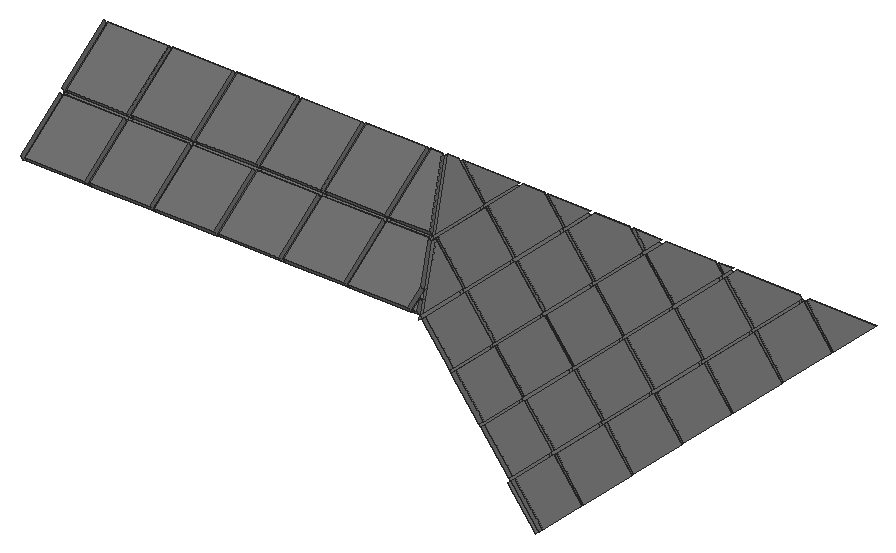
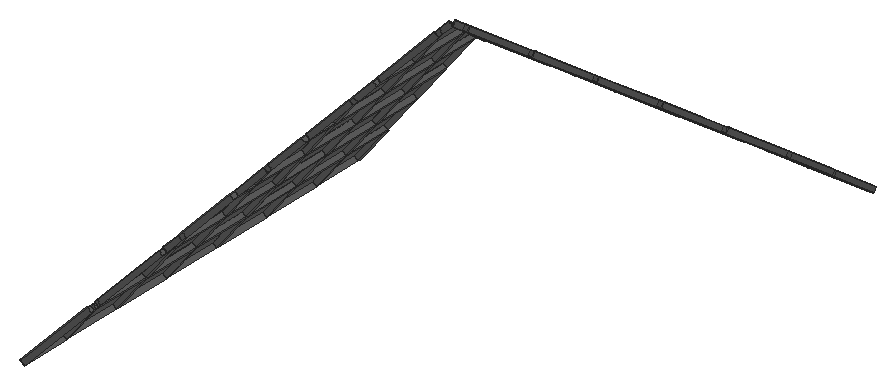
# SketchUp Ruby script. Lengths in inches.
U = 1.inch
M = Sketchup.active_model
def pt(a) = Geom::Point3d.new(a.map { |v| v * U })
def face(e, loops, mat)
  f = e.add_face(loops[0].map { |a| pt(a) })
  loops[1..].each { |l| e.add_face(l.map { |a| pt(a) }).erase! }
  f.material = f.back_material = mat if mat
  f
end
# faces: each face lists its corners as indices into pts; further lists are holes
def faces(e, pts, list, mat = nil) = list.each { |f| face(e, (f[0].is_a?(Array) ? f : [f]).map { |l| l.map { |i| pts[i] } }, mat) }
# xy, xz, yz: faces in a plane at the given z, y or x. An outline is a flat list of corners, or four numbers for a rectangle; further outlines are holes
def ring(l) = l.size == 4 ? [[l[0], l[1]], [l[2], l[1]], [l[2], l[3]], [l[0], l[3]]] : l.each_slice(2).to_a
def flat(e, list, mat, &to3) = list.each { |f| face(e, (f[0].is_a?(Array) ? f : [f]).map { |l| ring(l).map { |u, v| to3.(u, v) } }, mat) }
def xy(e, z, list, mat = nil) = flat(e, list, mat) { |x, y| [x, y, z] }
def xz(e, y, list, mat = nil) = flat(e, list, mat) { |x, z| [x, y, z] }
def yz(e, x, list, mat = nil) = flat(e, list, mat) { |y, z| [x, y, z] }
def lines(e, pts, list) = list.each { |a, b| e.add_line(pt(pts[a]), pt(pts[b])) }
# prism: a flat outline (further loops are holes) pulled along v
def prism(e, loops, v, mat = nil)
  f = face(e, loops, mat); d = Geom::Vector3d.new(v.map { |x| x * U })
  f.pushpull(f.normal.samedirection?(d) ? d.length : -d.length)
end
def box(e, o, s, mat = nil) = prism(e, [[o, [o[0] + s[0], o[1], o[2]], [o[0] + s[0], o[1] + s[1], o[2]], [o[0], o[1] + s[1], o[2]]]], [0, 0, s[2]], mat)
def at(x, y, z, deg = 0) = Geom::Transformation.translation(pt([x, y, z])) * Geom::Transformation.rotation(ORIGIN, Z_AXIS, deg.degrees)
def axes(o, x, y, z) = Geom::Transformation.new([*x, 0, *y, 0, *z, 0, *pt(o).to_a, 1])
def part(name) = M.definitions.add(name)
# library, detail: a bought-in or finely detailed component or shape, given as its bounding box
def library(name, o, s) = part(name).tap { |d| box(d.entities, o, s) }
def detail(e, o, s) = box(e.add_group.entities, o, s)
def put(e, d, t, mat = nil) = e.add_instance(d, t).tap { |i| i.material = mat if mat }
def group(e, t, mat = nil) = e.add_group.tap { |g| g.transformation = t; g.material = mat if mat }.entities
root = M.entities
M.materials.add("[Color M05]").color = [114, 114, 114]
xz(root,415.43,[[759.6,444.64,761.18,445.87,750.86,459.15,749.28,457.92],[748.6,458.81,750.18,460.04,739.86,473.32,738.28,472.1],[737.59,472.98,739.17,474.21,728.85,487.49,727.27,486.27],[726.58,487.15,728.16,488.38,717.84,501.67,716.26,500.4375]],"[Color M05]")
xz(root,433.59,[[759.6,444.64,749.28,457.92,750.86,459.15,761.18,445.87],[748.6,458.81,738.28,472.1,739.86,473.32,750.18,460.04],[737.59,472.98,727.27,486.27,728.85,487.49,739.17,474.21],[726.58,487.15,716.26,500.4375,717.84,501.67,728.16,488.38],[715.58,501.32,705.26,514.61,706.84,515.84,717.16,502.55]],"[Color M05]")
xz(root,434.8,[[759.6,444.64,761.18,445.87,750.86,459.15,749.28,457.92],[748.6,458.81,750.18,460.04,739.86,473.32,738.28,472.1],[737.59,472.98,739.17,474.21,728.85,487.49,727.27,486.27],[726.58,487.15,728.16,488.38,717.84,501.67,716.26,500.4375],[715.58,501.32,717.16,502.55,706.84,515.84,705.26,514.61]],"[Color M05]")
xz(root,456.8,[[759.6,444.64,749.28,457.92,750.86,459.15,761.18,445.87],[748.6,458.81,738.28,472.1,739.86,473.32,750.18,460.04],[737.59,472.98,727.27,486.27,728.85,487.49,739.17,474.21],[726.58,487.15,716.26,500.4375,717.84,501.67,728.16,488.38],[715.58,501.32,705.26,514.61,706.84,515.84,717.16,502.55],
  [704.57,515.5,695.0625,527.74,696.64,528.97,706.15,516.72]],"[Color M05]")
xz(root,458.01,[[759.6,444.64,761.18,445.87,750.86,459.15,749.28,457.92],[748.6,458.81,750.18,460.04,739.86,473.32,738.28,472.1],[737.59,472.98,739.17,474.21,728.85,487.49,727.27,486.27],[726.58,487.15,728.16,488.38,717.84,501.67,716.26,500.4375],[715.58,501.32,717.16,502.55,706.84,515.84,705.26,514.61],
  [704.57,515.5,706.15,516.72,697.33,528.08,695.75,526.85]],"[Color M05]")
xz(root,480.02,[[759.6,444.64,749.28,457.92,750.86,459.15,761.18,445.87],[748.6,458.81,738.28,472.1,739.86,473.32,750.18,460.04],[737.59,472.98,727.27,486.27,728.85,487.49,739.17,474.21],[726.58,487.15,716.26,500.4375,717.84,501.67,728.16,488.38],[715.58,501.32,708.25,510.76,709.83,511.98,717.16,502.55]],"[Color M05]")
xz(root,481.23,[[759.6,444.64,761.18,445.87,750.86,459.15,749.28,457.92],[748.6,458.81,750.18,460.04,739.86,473.32,738.28,472.1],[737.59,472.98,739.17,474.21,728.85,487.49,727.27,486.27],[726.58,487.15,728.16,488.38,717.84,501.67,716.26,500.4375],[715.58,501.32,717.16,502.55,710.52,511.1,708.94,509.87]],"[Color M05]")
xz(root,503.23,[[759.6,444.64,749.28,457.92,750.86,459.15,761.18,445.87],[748.6,458.81,738.28,472.1,739.86,473.32,750.18,460.04],[737.59,472.98,727.27,486.27,728.85,487.49,739.17,474.21],[726.58,487.15,721.44,493.77,723.02,495,728.16,488.38]],"[Color M05]")
xz(root,504.44,[[759.6,444.64,761.18,445.87,750.86,459.15,749.28,457.92],[748.6,458.81,750.18,460.04,739.86,473.32,738.28,472.1],[737.59,472.98,739.17,474.21,728.85,487.49,727.27,486.27],[726.58,487.15,728.16,488.38,723.71,494.11,722.13,492.89]],"[Color M05]")
xz(root,526.45,[[759.6,444.64,749.28,457.92,750.86,459.15,761.18,445.87],[748.6,458.81,738.28,472.1,739.86,473.32,750.18,460.04],[737.59,472.98,734.63,476.79,736.21,478.01,739.17,474.21]],"[Color M05]")
xz(root,527.66,[[759.6,444.64,761.18,445.87,750.86,459.15,749.28,457.92],[748.6,458.81,750.18,460.04,739.86,473.32,738.28,472.1],[737.59,472.98,739.17,474.21,736.9,477.13,735.32,475.9]],"[Color M05]")
xz(root,549.66,[[759.6,444.64,749.28,457.92,750.86,459.15,761.18,445.87],[748.6,458.81,747.82,459.8,749.4,461.03,750.18,460.04]],"[Color M05]")
xz(root,550.86,[[759.6,444.64,761.18,445.87,750.86,459.15,749.28,457.92]],"[Color M05]")
yz(root,568.12,[[415.43,501.32,433.59,514.61,432.41,516.22,414.25,502.9375],[434.8,515.5,454.17,529.67,452.99,531.28,433.62,517.11]],"[Color M05]")
yz(root,569.62,[[415.43,501.32,414.25,502.9375,432.41,516.22,433.59,514.61],[434.8,515.5,433.62,517.11,452.99,531.28,454.17,529.67]],"[Color M05]")
yz(root,592.12,[[415.43,501.32,433.59,514.61,432.41,516.22,414.25,502.9375],[434.8,515.5,454.17,529.67,452.99,531.28,433.62,517.11]],"[Color M05]")
yz(root,593.62,[[415.43,501.32,414.25,502.9375,432.41,516.22,433.59,514.61],[434.8,515.5,433.62,517.11,452.99,531.28,454.17,529.67]],"[Color M05]")
yz(root,617.62,[[415.43,501.32,414.25,502.9375,432.41,516.22,433.59,514.61],[434.8,515.5,433.62,517.11,452.99,531.28,454.17,529.67]],"[Color M05]")
yz(root,640.12,[[415.43,501.32,433.59,514.61,432.41,516.22,414.25,502.9375],[434.8,515.5,454.17,529.67,452.99,531.28,433.62,517.11]],"[Color M05]")
yz(root,641.62,[[415.43,501.32,414.25,502.9375,432.41,516.22,433.59,514.61],[434.8,515.5,433.62,517.11,452.99,531.28,454.17,529.67]],"[Color M05]")
yz(root,664.12,[[415.43,501.32,433.59,514.61,432.41,516.22,414.25,502.9375],[434.8,515.5,454.17,529.67,452.99,531.28,433.62,517.11]],"[Color M05]")
yz(root,665.62,[[415.43,501.32,414.25,502.9375,432.41,516.22,433.59,514.61],[434.8,515.5,433.62,517.11,452.99,531.28,454.17,529.67]],"[Color M05]")
yz(root,688.12,[[415.43,501.32,433.59,514.61,432.41,516.22,414.25,502.9375],[434.8,515.5,454.17,529.67,452.99,531.28,433.62,517.11]],"[Color M05]")
yz(root,689.62,[[415.43,501.32,414.25,502.9375,432.41,516.22,433.59,514.61],[434.8,515.5,433.62,517.11,452.99,531.28,454.17,529.67]],"[Color M05]")
yz(root,712.12,[[415.43,501.32,421.51,505.77,420.33,507.39,414.25,502.9375]],"[Color M05]")
yz(root,713.62,[[415.43,501.32,414.25,502.9375,417.69,505.45,418.87,503.84]],"[Color M05]")
p = [[759.6,414.22,444.64],[759.6,415.43,444.64],[749.28,415.43,457.92],[749.28,414.22,457.92],[759.6,433.59,444.64],[761.18,433.59,445.87],
  [761.18,415.43,445.87],[759.6,434.8,444.64],[749.28,434.8,457.92],[749.28,433.59,457.92],[759.6,456.8,444.64],[761.18,456.8,445.87],
  [761.18,434.8,445.87],[759.6,458.01,444.64],[749.28,458.01,457.92],[749.28,456.8,457.92],[759.6,480.02,444.64],[761.18,480.02,445.87],
  [761.18,458.01,445.87],[759.6,481.23,444.64],[749.28,481.23,457.92],[749.28,480.02,457.92],[759.6,503.23,444.64],[761.18,503.23,445.87],
  [761.18,481.23,445.87],[759.6,504.44,444.64],[749.28,504.44,457.92],[749.28,503.23,457.92],[759.6,526.45,444.64],[761.18,526.45,445.87],
  [761.18,504.44,445.87],[759.6,527.66,444.64],[749.28,527.66,457.92],[749.28,526.45,457.92],[759.6,549.66,444.64],[761.18,549.66,445.87],
  [761.18,527.66,445.87],[759.6,550.86,444.64],[749.28,550.86,457.92],[749.28,549.66,457.92],[759.6,570.39,444.64],[761.18,570.39,445.87],
  [761.18,550.86,445.87],[749.28,552.23,457.92],[750.86,552.23,459.15],[750.86,433.59,459.15],[750.86,415.43,459.15],[750.86,456.8,459.15],
  [750.86,434.8,459.15],[750.86,480.02,459.15],[750.86,458.01,459.15],[750.86,503.23,459.15],[750.86,481.23,459.15],[750.86,526.45,459.15],
  [750.86,504.44,459.15],[750.86,549.66,459.15],[750.86,527.66,459.15],[750.86,550.86,459.15],[748.6,433.59,458.81],[748.6,415.43,458.81],
  [748.6,434.8,458.81],[748.6,456.8,458.81],[748.6,458.01,458.81],[748.6,480.02,458.81],[748.6,481.23,458.81],[748.6,503.23,458.81],
  [748.6,504.44,458.81],[748.6,526.45,458.81],[748.6,527.66,458.81],[748.6,549.66,458.81],[748.6,550.86,458.81],[748.6,551.02,458.81],
  [750.18,433.59,460.04],[750.18,415.43,460.04],[738.28,434.8,472.1],[738.28,433.59,472.1],[750.18,456.8,460.04],[750.18,434.8,460.04],
  [738.28,458.01,472.1],[738.28,456.8,472.1],[750.18,480.02,460.04],[750.18,458.01,460.04],[738.28,481.23,472.1],[738.28,480.02,472.1],
  [750.18,503.23,460.04],[750.18,481.23,460.04],[738.28,504.44,472.1],[738.28,503.23,472.1],[750.18,526.45,460.04],[750.18,504.44,460.04],
  [738.28,527.66,472.1],[738.28,526.45,472.1],[750.18,549.66,460.04],[750.18,527.66,460.04],[748.5,550.86,458.93],[747.82,549.66,459.8],
  [738.28,532.86,472.1],[739.86,532.86,473.32],[749.4,549.66,461.03],[739.86,433.59,473.32],[739.86,415.43,473.32],[739.86,456.8,473.32],
  [739.86,434.8,473.32],[739.86,480.02,473.32],[739.86,458.01,473.32],[739.86,503.23,473.32],[739.86,481.23,473.32],[739.86,526.45,473.32],
  [739.86,504.44,473.32],[739.86,527.66,473.32],[738.28,415.43,472.1],[737.59,433.59,472.98],[737.59,415.43,472.98],[737.59,434.8,472.98],
  [737.59,456.8,472.98],[737.59,458.01,472.98],[737.59,480.02,472.98],[737.59,481.23,472.98],[737.59,503.23,472.98],[737.59,504.44,472.98],
  [737.59,526.45,472.98],[737.59,527.66,472.98],[737.59,531.65,472.98],[739.17,433.59,474.21],[739.17,415.43,474.21],[727.27,434.8,486.27],
  [727.27,433.59,486.27],[739.17,456.8,474.21],[739.17,434.8,474.21],[727.27,458.01,486.27],[727.27,456.8,486.27],[739.17,480.02,474.21],
  [739.17,458.01,474.21],[727.27,481.23,486.27],[727.27,480.02,486.27],[739.17,503.23,474.21],[739.17,481.23,474.21],[727.27,504.44,486.27],
  [727.27,503.23,486.27],[739.17,526.45,474.21],[739.17,504.44,474.21],[735.32,527.66,475.9],[734.63,526.45,476.79],[736.9,527.66,477.13],
  [739.17,531.65,474.21],[739.17,527.66,474.21],[728.85,433.59,487.49],[728.85,415.43,487.49],[728.85,456.8,487.49],[728.85,434.8,487.49],
  [728.85,480.02,487.49],[728.85,458.01,487.49],[728.85,503.23,487.49],[728.85,481.23,487.49],[736.21,526.45,478.01],[728.85,513.49,487.49],
  [728.85,504.44,487.49],[727.27,513.49,486.27],[727.27,415.43,486.27],[726.58,433.59,487.15],[726.58,415.43,487.15],[726.58,434.8,487.15],
  [726.58,456.8,487.15],[726.58,458.01,487.15],[726.58,480.02,487.15],[726.58,481.23,487.15],[726.58,503.23,487.15],[726.58,504.44,487.15],
  [726.58,512.28,487.15],[728.16,433.59,488.38],[728.16,415.43,488.38],[716.26,434.8,500.4375],[716.26,433.59,500.4375],[728.16,456.8,488.38],
  [728.16,434.8,488.38],[716.26,458.01,500.4375],[716.26,456.8,500.4375],[728.16,480.02,488.38],[728.16,458.01,488.38],[716.26,481.23,500.4375],
  [716.26,480.02,500.4375],[728.16,503.23,488.38],[728.16,481.23,488.38],[722.13,504.44,492.89],[721.44,503.23,493.77],[723.71,504.44,494.11],
  [728.16,512.28,488.38],[728.16,504.44,488.38],[717.84,433.59,501.67],[717.84,415.43,501.67],[717.84,456.8,501.67],[717.84,434.8,501.67],
  [717.84,480.02,501.67],[717.84,458.01,501.67],[723.02,503.23,495],[717.84,494.12,501.67],[717.84,481.23,501.67],[716.26,494.12,500.4375],
  [716.26,414.22,500.4375],[716.26,415.43,500.4375],[715.58,415.43,501.32],[715.58,433.59,501.32],[715.58,434.8,501.32],[715.58,456.8,501.32],
  [715.58,458.01,501.32],[715.58,480.02,501.32],[715.58,481.23,501.32],[715.58,492.91,501.32],[569.62,415.43,501.32],[592.12,415.43,501.32],
  [592.12,414.25,502.9375],[569.62,414.25,502.9375],[593.62,415.43,501.32],[616.13,415.43,501.32],[616.13,414.25,502.9375],[593.62,414.25,502.9375],
  [616.125,433.59,514.61],[616.125,432.41,516.22],[617.62,415.43,501.32],[640.12,415.43,501.32],[640.12,414.25,502.9375],[617.62,414.25,502.9375],
  [641.62,415.43,501.32],[664.12,415.43,501.32],[664.12,414.25,502.9375],[641.62,414.25,502.9375],[665.62,415.43,501.32],[688.12,415.43,501.32],
  [688.12,414.25,502.9375],[665.62,414.25,502.9375],[689.62,415.43,501.32],[712.12,415.43,501.32],[712.12,414.25,502.9375],[689.62,414.25,502.9375],
  [713.62,415.43,501.32],[715.58,414.25,502.9375],[713.62,414.25,502.9375],[713.62,418.87,503.84],[713.62,417.69,505.45],[568.12,415.43,501.32],
  [569.62,433.59,514.61],[568.12,433.59,514.61],[593.62,433.59,514.61],[592.12,433.59,514.61],[617.62,433.59,514.61],[641.62,433.59,514.61],
  [640.12,433.59,514.61],[665.62,433.59,514.61],[664.12,433.59,514.61],[689.62,433.59,514.61],[688.12,433.59,514.61],[712.12,421.51,505.77],
  [717.16,415.43,502.55],[715.2,418.87,505.07],[717.16,433.59,502.55],[705.26,434.8,514.61],[705.26,433.59,514.61],[717.16,456.8,502.55],
  [717.16,434.8,502.55],[705.26,458.01,514.61],[705.26,456.8,514.61],[717.16,480.02,502.55],[717.16,458.01,502.55],[708.94,481.23,509.87],
  [708.25,480.02,510.76],[710.52,481.23,511.1],[717.16,492.91,502.55],[717.16,481.23,502.55],[706.84,433.59,515.84],[713.7,421.51,507],
  [706.84,456.8,515.84],[706.84,434.8,515.84],[709.83,480.02,511.98],[706.84,474.75,515.84],[706.84,458.01,515.84],[592.12,432.41,516.22],
  [569.62,432.41,516.22],[593.62,432.41,516.22],[640.12,432.41,516.22],[617.62,432.41,516.22],[664.12,432.41,516.22],[641.62,432.41,516.22],
  [688.12,432.41,516.22],[665.62,432.41,516.22],[712.12,420.33,507.39],[705.26,432.41,516.22],[689.62,432.41,516.22],[705.26,474.75,514.61],
  [569.62,434.8,515.5],[568.12,434.8,515.5],[592.12,434.8,515.5],[593.62,434.8,515.5],[616.125,434.8,515.5],[617.62,434.8,515.5],
  [640.12,434.8,515.5],[641.62,434.8,515.5],[664.12,434.8,515.5],[665.62,434.8,515.5],[688.12,434.8,515.5],[689.62,434.8,515.5],
  [704.57,434.8,515.5],[704.57,456.8,515.5],[704.57,458.01,515.5],[704.57,473.54,515.5],[592.12,433.62,517.11],[569.62,433.62,517.11],
  [616.125,433.62,517.11],[593.62,433.62,517.11],[616.12,454.17,529.67],[616.12,452.99,531.28],[640.12,433.62,517.11],[617.62,433.62,517.11],
  [664.12,433.62,517.11],[641.62,433.62,517.11],[688.12,433.62,517.11],[665.62,433.62,517.11],[704.57,433.62,517.11],[689.62,433.62,517.11],
  [693.5625,454.17,529.67],[693.5625,452.99,531.28],[569.62,454.17,529.67],[568.12,454.17,529.67],[593.62,454.17,529.67],[592.12,454.17,529.67],
  [617.62,454.17,529.67],[641.62,454.17,529.67],[640.12,454.17,529.67],[665.62,454.17,529.67],[664.12,454.17,529.67],[689.62,454.17,529.67],
  [688.12,454.17,529.67],[706.15,434.8,516.72],[695.14,454.17,530.89],[706.15,456.8,516.72],[695.75,458.01,526.85],[695.0625,456.8,527.74],
  [697.33,458.01,528.08],[706.15,473.54,516.72],[706.15,458.01,516.72],[696.64,456.8,528.97],[592.12,452.99,531.28],[569.62,452.99,531.28],
  [593.62,452.99,531.28],[640.12,452.99,531.28],[617.62,452.99,531.28],[664.12,452.99,531.28],[641.62,452.99,531.28],[688.12,452.99,531.28],
  [665.62,452.99,531.28],[689.62,452.99,531.28]]
faces(root,p,[[0,1,2,3],[1,4,5,6],[4,7,8,9],[7,10,11,12],[10,13,14,15],[13,16,17,18],[16,19,20,21],[19,22,23,24],
  [22,25,26,27],[25,28,29,30],[28,31,32,33],[31,34,35,36],[34,37,38,39],[37,40,41,42],[40,43,44,41],[6,5,45,46],
  [12,11,47,48],[18,17,49,50],[24,23,51,52],[30,29,53,54],[36,35,55,56],[44,57,42,41],[2,9,58,59],[9,2,46,45],
  [9,8,60,58],[8,15,61,60],[15,8,48,47],[15,14,62,61],[14,21,63,62],[21,14,50,49],[21,20,64,63],[20,27,65,64],
  [27,20,52,51],[27,26,66,65],[26,33,67,66],[33,26,54,53],[33,32,68,67],[32,39,69,68],[39,32,56,55],[39,38,70,69],
  [71,70,38,43],[43,38,57,44],[59,58,72,73],[58,60,74,75],[60,61,76,77],[61,62,78,79],[62,63,80,81],[63,64,82,83],
  [64,65,84,85],[65,66,86,87],[66,67,88,89],[67,68,90,91],[68,69,92,93],[69,70,94,95],[71,94,70],[95,96,97,98],
  [73,72,99,100],[77,76,101,102],[81,80,103,104],[85,84,105,106],[89,88,107,108],[93,92,98,97,109],[110,75,111,112],[75,110,100,99],
  [75,74,113,111],[74,79,114,113],[79,74,102,101],[79,78,115,114],[78,83,116,115],[83,78,104,103],[83,82,117,116],[82,87,118,117],
  [87,82,106,105],[87,86,119,118],[86,91,120,119],[91,86,108,107],[91,90,121,120],[122,121,90,96],[96,90,109,97],[112,111,123,124],
  [111,113,125,126],[113,114,127,128],[114,115,129,130],[115,116,131,132],[116,117,133,134],[117,118,135,136],[118,119,137,138],[119,120,139,140],
  [120,121,141,142],[122,141,143,144],[121,122,144,145],[124,123,146,147],[128,127,148,149],[132,131,150,151],[136,135,152,153],[140,139,154,155,156],
  [144,143,145],[142,157,155,154],[158,126,159,160],[126,158,147,146],[126,125,161,159],[125,130,162,161],[130,125,149,148],[130,129,163,162],
  [129,134,164,163],[134,129,151,150],[134,133,165,164],[133,138,166,165],[138,133,153,152],[138,137,167,166],[168,167,137,157],[157,137,156,155],
  [160,159,169,170],[159,161,171,172],[161,162,173,174],[162,163,175,176],[163,164,177,178],[164,165,179,180],[165,166,181,182],[166,167,183,184],
  [168,183,185,186],[167,168,186,187],[170,169,188,189],[174,173,190,191],[178,177,192,193],[182,181,194,195,196],[186,185,187],[184,197,195,194],
  [198,199,200],[199,172,201,200],[172,199,189,188],[172,171,202,201],[171,176,203,202],[176,171,191,190],[176,175,204,203],[175,180,205,204],
  [180,175,193,192],[180,179,206,205],[207,206,179,197],[197,179,196,195],[208,209,210,211],[212,213,214,215],[213,216,217,214],[218,219,220,221],
  [222,223,224,225],[226,227,228,229],[230,231,232,233],[234,200,235,236],[200,237,238,235],[239,208,240,241],[209,212,242,243],[213,218,244,216],
  [219,222,245,246],[223,226,247,248],[227,230,249,250],[231,234,237,251],[237,200,252,253],[200,201,254,252],[201,202,255,256],[202,203,257,258],
  [203,204,259,260],[204,205,261,262],[205,206,263,264],[207,263,265,266],[206,207,266,267],[252,254,268,269,253],[258,257,270,271],[262,261,272,273,274],
  [266,265,267],[211,210,275,276],[215,214,217,277],[221,220,278,279],[225,224,280,281],[229,228,282,283],[233,232,284,285,286],[235,238,236],
  [251,237,253,269],[251,256,285,284],[256,251,269,268],[264,287,273,272],[243,240,276,275],[216,242,277,217],[246,244,279,278],[248,245,281,280],
  [250,247,283,282],[256,249,286,285],[241,240,288,289],[240,243,290,288],[243,242,291,290],[242,216,292,291],[216,244,293,292],[244,246,294,293],
  [246,245,295,294],[245,248,296,295],[248,247,297,296],[247,250,298,297],[250,249,299,298],[300,299,249,256],[256,255,300],[255,260,301,300],
  [260,255,271,270],[260,259,302,301],[303,302,259,287],[287,259,274,273],[288,290,304,305],[291,292,306,307],[292,308,309,306],[293,294,310,311],
  [295,296,312,313],[297,298,314,315],[299,300,316,317],[300,318,319,316],[289,288,320,321],[290,291,322,323],[292,293,324,308],[294,295,325,326],
  [296,297,327,328],[298,299,329,330],[318,300,331,332],[300,301,333,331],[301,302,334,335],[303,334,336,337],[302,303,337,338],[331,333,339,332],
  [337,336,338],[305,304,340,341],[307,306,309,342],[311,310,343,344],[313,312,345,346],[315,314,347,348],[319,349,317,316],[335,318,332,339],
  [323,320,341,340],[308,322,342,309],[326,324,344,343],[328,325,346,345],[330,327,348,347],[318,329,349,319]],"[Color M05]")
